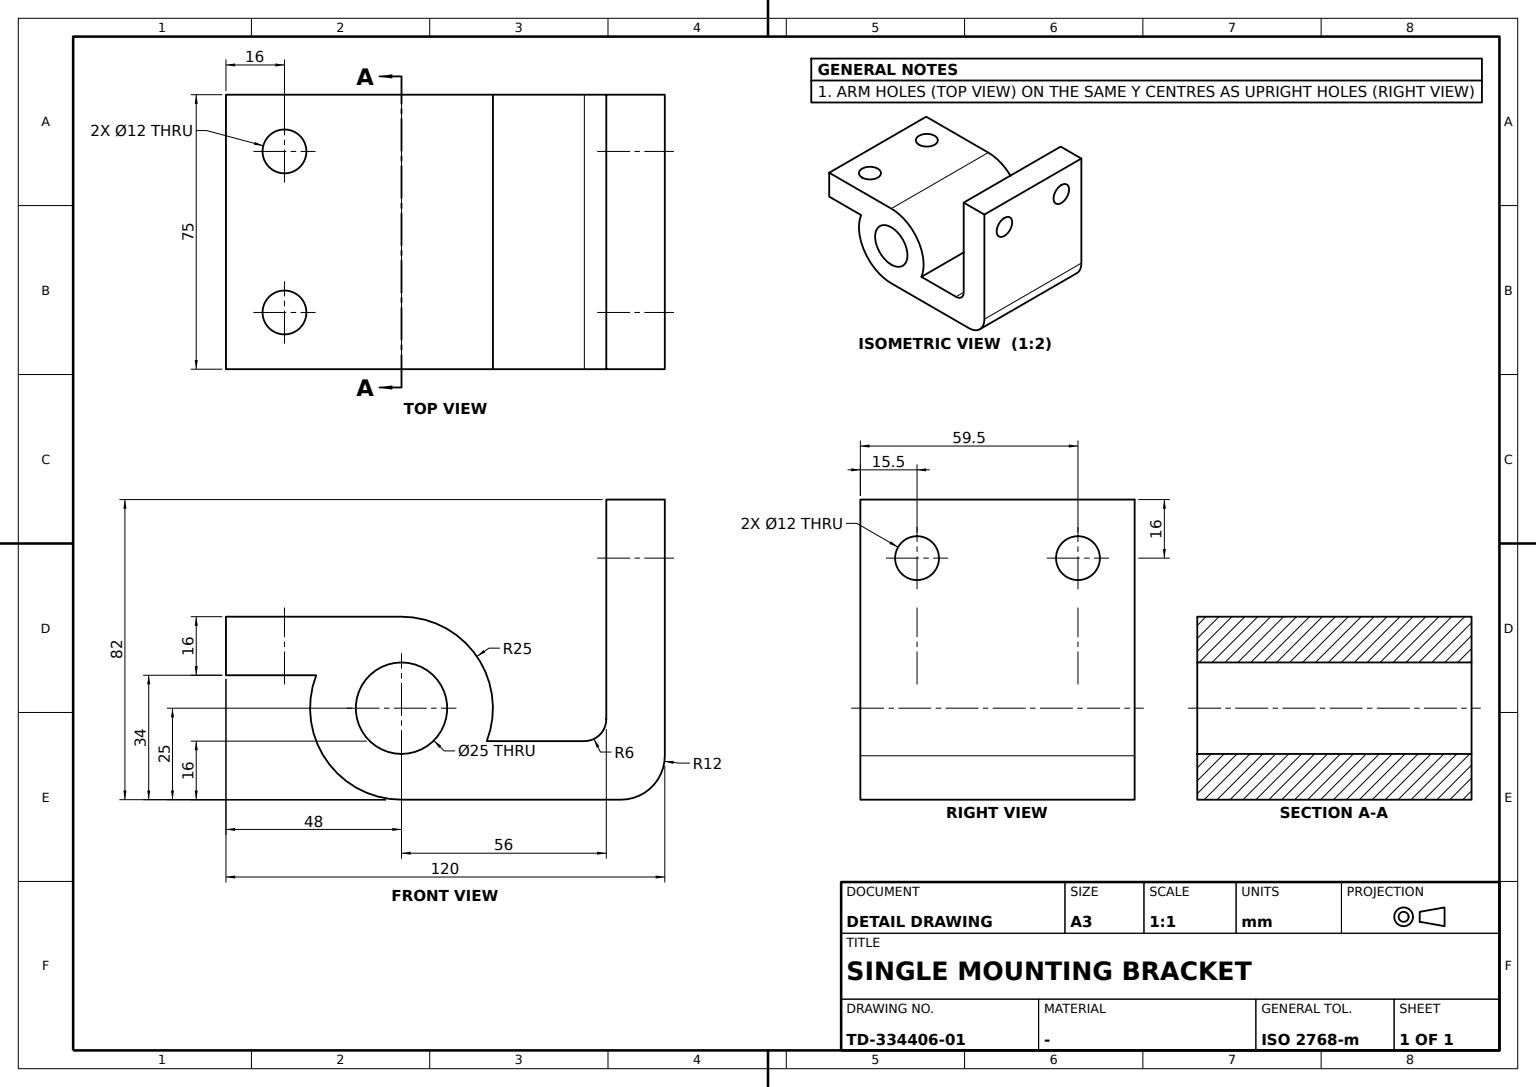
ISO-10303-21;
HEADER;
FILE_DESCRIPTION((''),'2;1');
FILE_NAME('','',(''),(''),'','','');
FILE_SCHEMA(('AUTOMOTIVE_DESIGN'));
ENDSEC;
DATA;
#1=APPLICATION_CONTEXT('');
#2=PRODUCT_CONTEXT('',#1,'mechanical');
#3=PRODUCT('','','',(#2));
#4=PRODUCT_DEFINITION_FORMATION('','',#3);
#5=PRODUCT_DEFINITION_CONTEXT('',#1,'design');
#6=PRODUCT_DEFINITION('','',#4,#5);
#7=PRODUCT_DEFINITION_SHAPE('','',#6);
#8=(LENGTH_UNIT()NAMED_UNIT(*)SI_UNIT(.MILLI.,.METRE.));
#9=(NAMED_UNIT(*)PLANE_ANGLE_UNIT()SI_UNIT($,.RADIAN.));
#10=(NAMED_UNIT(*)SI_UNIT($,.STERADIAN.)SOLID_ANGLE_UNIT());
#11=UNCERTAINTY_MEASURE_WITH_UNIT(LENGTH_MEASURE(0.005),#8,'distance_accuracy_value','');
#12=(GEOMETRIC_REPRESENTATION_CONTEXT(3)GLOBAL_UNCERTAINTY_ASSIGNED_CONTEXT((#11))GLOBAL_UNIT_ASSIGNED_CONTEXT((#8,#9,#10))REPRESENTATION_CONTEXT('',''));
#13=CARTESIAN_POINT('',(-37.5,-23.323808,9.));
#14=VERTEX_POINT('',#13);
#15=CARTESIAN_POINT('',(-37.5,0.,-25.));
#16=VERTEX_POINT('',#15);
#17=CARTESIAN_POINT('',(-37.5,0.,0.));
#18=DIRECTION('',(1.,0.,0.));
#19=DIRECTION('',(0.,0.,-1.));
#20=AXIS2_PLACEMENT_3D('',#17,#18,#19);
#21=CIRCLE('',#20,25.);
#22=EDGE_CURVE('',#14,#16,#21,.T.);
#23=ORIENTED_EDGE('',*,*,#22,.T.);
#24=CARTESIAN_POINT('',(37.5,0.,-25.));
#25=VERTEX_POINT('',#24);
#26=CARTESIAN_POINT('',(0.,0.,-25.));
#27=VECTOR('',#18,1000.);
#28=LINE('',#26,#27);
#29=EDGE_CURVE('',#16,#25,#28,.T.);
#30=ORIENTED_EDGE('',*,*,#29,.T.);
#31=CARTESIAN_POINT('',(37.5,-23.323808,9.));
#32=VERTEX_POINT('',#31);
#33=CARTESIAN_POINT('',(37.5,0.,0.));
#34=AXIS2_PLACEMENT_3D('',#33,#18,#19);
#35=CIRCLE('',#34,25.);
#36=EDGE_CURVE('',#32,#25,#35,.T.);
#37=ORIENTED_EDGE('',*,*,#36,.F.);
#38=LINE('',#13,#27);
#39=EDGE_CURVE('',#14,#32,#38,.T.);
#40=ORIENTED_EDGE('',*,*,#39,.F.);
#41=EDGE_LOOP('',(#23,#30,#37,#40));
#42=FACE_BOUND('',#41,.T.);
#43=CARTESIAN_POINT('',(0.,0.,0.));
#44=DIRECTION('',(0.,1.,0.));
#45=AXIS2_PLACEMENT_3D('',#43,#18,#44);
#46=CYLINDRICAL_SURFACE('',#45,25.);
#47=ADVANCED_FACE('',(#42),#46,.T.);
#48=CARTESIAN_POINT('',(22.,56.,47.));
#49=VERTEX_POINT('',#48);
#50=CARTESIAN_POINT('',(22.,56.,41.));
#51=DIRECTION('',(0.,0.,1.));
#52=AXIS2_PLACEMENT_3D('',#50,#44,#51);
#53=CIRCLE('',#52,6.);
#54=EDGE_CURVE('',#49,#49,#53,.T.);
#55=ORIENTED_EDGE('',*,*,#54,.F.);
#56=EDGE_LOOP('',(#55));
#57=FACE_BOUND('',#56,.T.);
#58=CARTESIAN_POINT('',(22.,72.,35.));
#59=VERTEX_POINT('',#58);
#60=CARTESIAN_POINT('',(22.,72.,41.));
#61=DIRECTION('',(0.,-1.,0.));
#62=AXIS2_PLACEMENT_3D('',#60,#61,#19);
#63=CIRCLE('',#62,6.);
#64=EDGE_CURVE('',#59,#59,#63,.F.);
#65=ORIENTED_EDGE('',*,*,#64,.T.);
#66=EDGE_LOOP('',(#65));
#67=FACE_BOUND('',#66,.T.);
#68=CARTESIAN_POINT('',(22.,53.25,41.));
#69=DIRECTION('',(-1.,0.,0.));
#70=AXIS2_PLACEMENT_3D('',#68,#44,#69);
#71=CYLINDRICAL_SURFACE('',#70,6.);
#72=ADVANCED_FACE('',(#57,#67),#71,.F.);
#73=CARTESIAN_POINT('',(-37.5,0.,25.));
#74=VERTEX_POINT('',#73);
#75=CARTESIAN_POINT('',(37.5,0.,25.));
#76=VERTEX_POINT('',#75);
#77=CARTESIAN_POINT('',(0.,0.,25.));
#78=LINE('',#77,#27);
#79=EDGE_CURVE('',#74,#76,#78,.T.);
#80=ORIENTED_EDGE('',*,*,#79,.T.);
#81=CARTESIAN_POINT('',(37.5,23.323808,-9.));
#82=VERTEX_POINT('',#81);
#83=EDGE_CURVE('',#82,#76,#35,.T.);
#84=ORIENTED_EDGE('',*,*,#83,.F.);
#85=CARTESIAN_POINT('',(-37.5,23.323808,-9.));
#86=VERTEX_POINT('',#85);
#87=LINE('',#85,#27);
#88=EDGE_CURVE('',#86,#82,#87,.T.);
#89=ORIENTED_EDGE('',*,*,#88,.F.);
#90=EDGE_CURVE('',#86,#74,#21,.T.);
#91=ORIENTED_EDGE('',*,*,#90,.T.);
#92=EDGE_LOOP('',(#80,#84,#89,#91));
#93=FACE_BOUND('',#92,.T.);
#94=ADVANCED_FACE('',(#93),#46,.T.);
#95=CARTESIAN_POINT('',(37.5,0.,-12.5));
#96=VERTEX_POINT('',#95);
#97=CIRCLE('',#34,12.5);
#98=EDGE_CURVE('',#96,#96,#97,.T.);
#99=ORIENTED_EDGE('',*,*,#98,.T.);
#100=EDGE_LOOP('',(#99));
#101=FACE_BOUND('',#100,.T.);
#102=CARTESIAN_POINT('',(-37.5,0.,-12.5));
#103=VERTEX_POINT('',#102);
#104=CIRCLE('',#20,12.5);
#105=EDGE_CURVE('',#103,#103,#104,.T.);
#106=ORIENTED_EDGE('',*,*,#105,.F.);
#107=EDGE_LOOP('',(#106));
#108=FACE_BOUND('',#107,.T.);
#109=CYLINDRICAL_SURFACE('',#45,12.5);
#110=ADVANCED_FACE('',(#101,#108),#109,.F.);
#111=CARTESIAN_POINT('',(16.,-32.,9.));
#112=VERTEX_POINT('',#111);
#113=CARTESIAN_POINT('',(22.,-32.,9.));
#114=AXIS2_PLACEMENT_3D('',#113,#19,#69);
#115=CIRCLE('',#114,6.);
#116=EDGE_CURVE('',#112,#112,#115,.T.);
#117=ORIENTED_EDGE('',*,*,#116,.F.);
#118=EDGE_LOOP('',(#117));
#119=FACE_BOUND('',#118,.T.);
#120=CARTESIAN_POINT('',(-28.,-32.,9.));
#121=VERTEX_POINT('',#120);
#122=CARTESIAN_POINT('',(-22.,-32.,9.));
#123=AXIS2_PLACEMENT_3D('',#122,#19,#69);
#124=CIRCLE('',#123,6.);
#125=EDGE_CURVE('',#121,#121,#124,.T.);
#126=ORIENTED_EDGE('',*,*,#125,.F.);
#127=EDGE_LOOP('',(#126));
#128=FACE_BOUND('',#127,.T.);
#129=CARTESIAN_POINT('',(37.5,-48.,9.));
#130=VERTEX_POINT('',#129);
#131=CARTESIAN_POINT('',(37.5,0.,9.));
#132=VECTOR('',#44,1000.);
#133=LINE('',#131,#132);
#134=EDGE_CURVE('',#130,#32,#133,.T.);
#135=ORIENTED_EDGE('',*,*,#134,.F.);
#136=CARTESIAN_POINT('',(-37.5,-48.,9.));
#137=VERTEX_POINT('',#136);
#138=CARTESIAN_POINT('',(0.,-48.,9.));
#139=LINE('',#138,#27);
#140=EDGE_CURVE('',#137,#130,#139,.T.);
#141=ORIENTED_EDGE('',*,*,#140,.F.);
#142=CARTESIAN_POINT('',(-37.5,0.,9.));
#143=LINE('',#142,#132);
#144=EDGE_CURVE('',#137,#14,#143,.T.);
#145=ORIENTED_EDGE('',*,*,#144,.T.);
#146=ORIENTED_EDGE('',*,*,#39,.T.);
#147=EDGE_LOOP('',(#135,#141,#145,#146));
#148=FACE_BOUND('',#147,.T.);
#149=AXIS2_PLACEMENT_3D('',#138,#19,#44);
#150=PLANE('',#149);
#151=ADVANCED_FACE('',(#119,#128,#148),#150,.T.);
#152=ORIENTED_EDGE('',*,*,#125,.T.);
#153=EDGE_LOOP('',(#152));
#154=FACE_BOUND('',#153,.T.);
#155=CARTESIAN_POINT('',(-16.,-32.,25.));
#156=VERTEX_POINT('',#155);
#157=CARTESIAN_POINT('',(-22.,-32.,25.));
#158=AXIS2_PLACEMENT_3D('',#157,#51,#18);
#159=CIRCLE('',#158,6.);
#160=EDGE_CURVE('',#156,#156,#159,.T.);
#161=ORIENTED_EDGE('',*,*,#160,.T.);
#162=EDGE_LOOP('',(#161));
#163=FACE_BOUND('',#162,.T.);
#164=CARTESIAN_POINT('',(-22.,-32.,6.25));
#165=AXIS2_PLACEMENT_3D('',#164,#51,#44);
#166=CYLINDRICAL_SURFACE('',#165,6.);
#167=ADVANCED_FACE('',(#154,#163),#166,.F.);
#168=CARTESIAN_POINT('',(-37.5,60.,-25.));
#169=VERTEX_POINT('',#168);
#170=CARTESIAN_POINT('',(37.5,60.,-25.));
#171=VERTEX_POINT('',#170);
#172=CARTESIAN_POINT('',(0.,60.,-25.));
#173=LINE('',#172,#27);
#174=EDGE_CURVE('',#169,#171,#173,.T.);
#175=ORIENTED_EDGE('',*,*,#174,.F.);
#176=CARTESIAN_POINT('',(-37.5,72.,-13.));
#177=VERTEX_POINT('',#176);
#178=CARTESIAN_POINT('',(-37.5,60.,-13.));
#179=AXIS2_PLACEMENT_3D('',#178,#18,#19);
#180=CIRCLE('',#179,12.);
#181=EDGE_CURVE('',#169,#177,#180,.T.);
#182=ORIENTED_EDGE('',*,*,#181,.T.);
#183=CARTESIAN_POINT('',(37.5,72.,-13.));
#184=VERTEX_POINT('',#183);
#185=CARTESIAN_POINT('',(0.,72.,-13.));
#186=LINE('',#185,#27);
#187=EDGE_CURVE('',#177,#184,#186,.T.);
#188=ORIENTED_EDGE('',*,*,#187,.T.);
#189=CARTESIAN_POINT('',(37.5,60.,-13.));
#190=AXIS2_PLACEMENT_3D('',#189,#18,#19);
#191=CIRCLE('',#190,12.);
#192=EDGE_CURVE('',#171,#184,#191,.T.);
#193=ORIENTED_EDGE('',*,*,#192,.F.);
#194=EDGE_LOOP('',(#175,#182,#188,#193));
#195=FACE_BOUND('',#194,.T.);
#196=CARTESIAN_POINT('',(0.,60.,-13.));
#197=AXIS2_PLACEMENT_3D('',#196,#18,#44);
#198=CYLINDRICAL_SURFACE('',#197,12.);
#199=ADVANCED_FACE('',(#195),#198,.T.);
#200=CARTESIAN_POINT('',(-22.,72.,35.));
#201=VERTEX_POINT('',#200);
#202=CARTESIAN_POINT('',(-22.,72.,41.));
#203=AXIS2_PLACEMENT_3D('',#202,#61,#19);
#204=CIRCLE('',#203,6.);
#205=EDGE_CURVE('',#201,#201,#204,.F.);
#206=ORIENTED_EDGE('',*,*,#205,.T.);
#207=EDGE_LOOP('',(#206));
#208=FACE_BOUND('',#207,.T.);
#209=CARTESIAN_POINT('',(-22.,56.,47.));
#210=VERTEX_POINT('',#209);
#211=CARTESIAN_POINT('',(-22.,56.,41.));
#212=AXIS2_PLACEMENT_3D('',#211,#44,#51);
#213=CIRCLE('',#212,6.);
#214=EDGE_CURVE('',#210,#210,#213,.T.);
#215=ORIENTED_EDGE('',*,*,#214,.F.);
#216=EDGE_LOOP('',(#215));
#217=FACE_BOUND('',#216,.T.);
#218=CARTESIAN_POINT('',(-22.,53.25,41.));
#219=AXIS2_PLACEMENT_3D('',#218,#44,#69);
#220=CYLINDRICAL_SURFACE('',#219,6.);
#221=ADVANCED_FACE('',(#208,#217),#220,.F.);
#222=ORIENTED_EDGE('',*,*,#144,.F.);
#223=CARTESIAN_POINT('',(-37.5,-48.,25.));
#224=VERTEX_POINT('',#223);
#225=CARTESIAN_POINT('',(-37.5,-48.,0.));
#226=VECTOR('',#19,1000.);
#227=LINE('',#225,#226);
#228=EDGE_CURVE('',#224,#137,#227,.T.);
#229=ORIENTED_EDGE('',*,*,#228,.F.);
#230=VECTOR('',#61,1000.);
#231=LINE('',#73,#230);
#232=EDGE_CURVE('',#74,#224,#231,.T.);
#233=ORIENTED_EDGE('',*,*,#232,.F.);
#234=ORIENTED_EDGE('',*,*,#90,.F.);
#235=CARTESIAN_POINT('',(-37.5,50.,-9.));
#236=VERTEX_POINT('',#235);
#237=CARTESIAN_POINT('',(-37.5,0.,-9.));
#238=LINE('',#237,#132);
#239=EDGE_CURVE('',#86,#236,#238,.T.);
#240=ORIENTED_EDGE('',*,*,#239,.T.);
#241=CARTESIAN_POINT('',(-37.5,56.,-3.));
#242=VERTEX_POINT('',#241);
#243=CARTESIAN_POINT('',(-37.5,50.,-3.));
#244=AXIS2_PLACEMENT_3D('',#243,#18,#19);
#245=CIRCLE('',#244,6.);
#246=EDGE_CURVE('',#236,#242,#245,.T.);
#247=ORIENTED_EDGE('',*,*,#246,.T.);
#248=CARTESIAN_POINT('',(-37.5,56.,57.));
#249=VERTEX_POINT('',#248);
#250=CARTESIAN_POINT('',(-37.5,56.,0.));
#251=VECTOR('',#51,1000.);
#252=LINE('',#250,#251);
#253=EDGE_CURVE('',#242,#249,#252,.T.);
#254=ORIENTED_EDGE('',*,*,#253,.T.);
#255=CARTESIAN_POINT('',(-37.5,72.,57.));
#256=VERTEX_POINT('',#255);
#257=CARTESIAN_POINT('',(-37.5,0.,57.));
#258=LINE('',#257,#132);
#259=EDGE_CURVE('',#249,#256,#258,.T.);
#260=ORIENTED_EDGE('',*,*,#259,.T.);
#261=CARTESIAN_POINT('',(-37.5,72.,0.));
#262=LINE('',#261,#226);
#263=EDGE_CURVE('',#256,#177,#262,.T.);
#264=ORIENTED_EDGE('',*,*,#263,.T.);
#265=ORIENTED_EDGE('',*,*,#181,.F.);
#266=LINE('',#15,#230);
#267=EDGE_CURVE('',#169,#16,#266,.T.);
#268=ORIENTED_EDGE('',*,*,#267,.T.);
#269=ORIENTED_EDGE('',*,*,#22,.F.);
#270=EDGE_LOOP('',(#222,#229,#233,#234,#240,#247,#254,#260,#264,#265,#268,#269));
#271=FACE_BOUND('',#270,.T.);
#272=ORIENTED_EDGE('',*,*,#105,.T.);
#273=EDGE_LOOP('',(#272));
#274=FACE_BOUND('',#273,.T.);
#275=AXIS2_PLACEMENT_3D('',#17,#18,#44);
#276=PLANE('',#275);
#277=ADVANCED_FACE('',(#271,#274),#276,.F.);
#278=CARTESIAN_POINT('',(28.,-32.,25.));
#279=VERTEX_POINT('',#278);
#280=CARTESIAN_POINT('',(22.,-32.,25.));
#281=AXIS2_PLACEMENT_3D('',#280,#51,#18);
#282=CIRCLE('',#281,6.);
#283=EDGE_CURVE('',#279,#279,#282,.T.);
#284=ORIENTED_EDGE('',*,*,#283,.T.);
#285=EDGE_LOOP('',(#284));
#286=FACE_BOUND('',#285,.T.);
#287=ORIENTED_EDGE('',*,*,#116,.T.);
#288=EDGE_LOOP('',(#287));
#289=FACE_BOUND('',#288,.T.);
#290=CARTESIAN_POINT('',(22.,-32.,6.25));
#291=AXIS2_PLACEMENT_3D('',#290,#51,#44);
#292=CYLINDRICAL_SURFACE('',#291,6.);
#293=ADVANCED_FACE('',(#286,#289),#292,.F.);
#294=CARTESIAN_POINT('',(37.5,56.,57.));
#295=VERTEX_POINT('',#294);
#296=CARTESIAN_POINT('',(37.5,72.,57.));
#297=VERTEX_POINT('',#296);
#298=CARTESIAN_POINT('',(37.5,0.,57.));
#299=LINE('',#298,#132);
#300=EDGE_CURVE('',#295,#297,#299,.T.);
#301=ORIENTED_EDGE('',*,*,#300,.T.);
#302=CARTESIAN_POINT('',(0.,72.,57.));
#303=LINE('',#302,#27);
#304=EDGE_CURVE('',#256,#297,#303,.T.);
#305=ORIENTED_EDGE('',*,*,#304,.F.);
#306=ORIENTED_EDGE('',*,*,#259,.F.);
#307=CARTESIAN_POINT('',(0.,56.,57.));
#308=LINE('',#307,#27);
#309=EDGE_CURVE('',#249,#295,#308,.T.);
#310=ORIENTED_EDGE('',*,*,#309,.T.);
#311=EDGE_LOOP('',(#301,#305,#306,#310));
#312=FACE_BOUND('',#311,.T.);
#313=AXIS2_PLACEMENT_3D('',#307,#19,#44);
#314=PLANE('',#313);
#315=ADVANCED_FACE('',(#312),#314,.F.);
#316=ORIENTED_EDGE('',*,*,#205,.F.);
#317=EDGE_LOOP('',(#316));
#318=FACE_BOUND('',#317,.T.);
#319=ORIENTED_EDGE('',*,*,#64,.F.);
#320=EDGE_LOOP('',(#319));
#321=FACE_BOUND('',#320,.T.);
#322=ORIENTED_EDGE('',*,*,#187,.F.);
#323=ORIENTED_EDGE('',*,*,#263,.F.);
#324=ORIENTED_EDGE('',*,*,#304,.T.);
#325=CARTESIAN_POINT('',(37.5,72.,0.));
#326=LINE('',#325,#226);
#327=EDGE_CURVE('',#297,#184,#326,.T.);
#328=ORIENTED_EDGE('',*,*,#327,.T.);
#329=EDGE_LOOP('',(#322,#323,#324,#328));
#330=FACE_BOUND('',#329,.T.);
#331=AXIS2_PLACEMENT_3D('',#302,#61,#19);
#332=PLANE('',#331);
#333=ADVANCED_FACE('',(#318,#321,#330),#332,.F.);
#334=ORIENTED_EDGE('',*,*,#98,.F.);
#335=EDGE_LOOP('',(#334));
#336=FACE_BOUND('',#335,.T.);
#337=LINE('',#24,#230);
#338=EDGE_CURVE('',#171,#25,#337,.T.);
#339=ORIENTED_EDGE('',*,*,#338,.F.);
#340=ORIENTED_EDGE('',*,*,#192,.T.);
#341=ORIENTED_EDGE('',*,*,#327,.F.);
#342=ORIENTED_EDGE('',*,*,#300,.F.);
#343=CARTESIAN_POINT('',(37.5,56.,-3.));
#344=VERTEX_POINT('',#343);
#345=CARTESIAN_POINT('',(37.5,56.,0.));
#346=LINE('',#345,#251);
#347=EDGE_CURVE('',#344,#295,#346,.T.);
#348=ORIENTED_EDGE('',*,*,#347,.F.);
#349=CARTESIAN_POINT('',(37.5,50.,-9.));
#350=VERTEX_POINT('',#349);
#351=CARTESIAN_POINT('',(37.5,50.,-3.));
#352=AXIS2_PLACEMENT_3D('',#351,#18,#19);
#353=CIRCLE('',#352,6.);
#354=EDGE_CURVE('',#350,#344,#353,.T.);
#355=ORIENTED_EDGE('',*,*,#354,.F.);
#356=CARTESIAN_POINT('',(37.5,0.,-9.));
#357=LINE('',#356,#132);
#358=EDGE_CURVE('',#82,#350,#357,.T.);
#359=ORIENTED_EDGE('',*,*,#358,.F.);
#360=ORIENTED_EDGE('',*,*,#83,.T.);
#361=CARTESIAN_POINT('',(37.5,-48.,25.));
#362=VERTEX_POINT('',#361);
#363=LINE('',#75,#230);
#364=EDGE_CURVE('',#76,#362,#363,.T.);
#365=ORIENTED_EDGE('',*,*,#364,.T.);
#366=CARTESIAN_POINT('',(37.5,-48.,0.));
#367=LINE('',#366,#226);
#368=EDGE_CURVE('',#362,#130,#367,.T.);
#369=ORIENTED_EDGE('',*,*,#368,.T.);
#370=ORIENTED_EDGE('',*,*,#134,.T.);
#371=ORIENTED_EDGE('',*,*,#36,.T.);
#372=EDGE_LOOP('',(#339,#340,#341,#342,#348,#355,#359,#360,#365,#369,#370,#371));
#373=FACE_BOUND('',#372,.T.);
#374=AXIS2_PLACEMENT_3D('',#33,#18,#44);
#375=PLANE('',#374);
#376=ADVANCED_FACE('',(#336,#373),#375,.T.);
#377=ORIENTED_EDGE('',*,*,#228,.T.);
#378=ORIENTED_EDGE('',*,*,#140,.T.);
#379=ORIENTED_EDGE('',*,*,#368,.F.);
#380=CARTESIAN_POINT('',(0.,-48.,25.));
#381=LINE('',#380,#27);
#382=EDGE_CURVE('',#224,#362,#381,.T.);
#383=ORIENTED_EDGE('',*,*,#382,.F.);
#384=EDGE_LOOP('',(#377,#378,#379,#383));
#385=FACE_BOUND('',#384,.T.);
#386=AXIS2_PLACEMENT_3D('',#380,#61,#19);
#387=PLANE('',#386);
#388=ADVANCED_FACE('',(#385),#387,.T.);
#389=ORIENTED_EDGE('',*,*,#29,.F.);
#390=ORIENTED_EDGE('',*,*,#267,.F.);
#391=ORIENTED_EDGE('',*,*,#174,.T.);
#392=ORIENTED_EDGE('',*,*,#338,.T.);
#393=EDGE_LOOP('',(#389,#390,#391,#392));
#394=FACE_BOUND('',#393,.T.);
#395=CARTESIAN_POINT('',(0.,72.,-25.));
#396=AXIS2_PLACEMENT_3D('',#395,#51,#61);
#397=PLANE('',#396);
#398=ADVANCED_FACE('',(#394),#397,.F.);
#399=ORIENTED_EDGE('',*,*,#214,.T.);
#400=EDGE_LOOP('',(#399));
#401=FACE_BOUND('',#400,.T.);
#402=ORIENTED_EDGE('',*,*,#253,.F.);
#403=CARTESIAN_POINT('',(0.,56.,-3.));
#404=LINE('',#403,#27);
#405=EDGE_CURVE('',#242,#344,#404,.T.);
#406=ORIENTED_EDGE('',*,*,#405,.T.);
#407=ORIENTED_EDGE('',*,*,#347,.T.);
#408=ORIENTED_EDGE('',*,*,#309,.F.);
#409=EDGE_LOOP('',(#402,#406,#407,#408));
#410=FACE_BOUND('',#409,.T.);
#411=ORIENTED_EDGE('',*,*,#54,.T.);
#412=EDGE_LOOP('',(#411));
#413=FACE_BOUND('',#412,.T.);
#414=CARTESIAN_POINT('',(0.,56.,-9.));
#415=AXIS2_PLACEMENT_3D('',#414,#44,#51);
#416=PLANE('',#415);
#417=ADVANCED_FACE('',(#401,#410,#413),#416,.F.);
#418=ORIENTED_EDGE('',*,*,#354,.T.);
#419=ORIENTED_EDGE('',*,*,#405,.F.);
#420=ORIENTED_EDGE('',*,*,#246,.F.);
#421=CARTESIAN_POINT('',(0.,50.,-9.));
#422=LINE('',#421,#27);
#423=EDGE_CURVE('',#236,#350,#422,.T.);
#424=ORIENTED_EDGE('',*,*,#423,.T.);
#425=EDGE_LOOP('',(#418,#419,#420,#424));
#426=FACE_BOUND('',#425,.T.);
#427=CARTESIAN_POINT('',(0.,50.,-3.));
#428=AXIS2_PLACEMENT_3D('',#427,#18,#19);
#429=CYLINDRICAL_SURFACE('',#428,6.);
#430=ADVANCED_FACE('',(#426),#429,.F.);
#431=ORIENTED_EDGE('',*,*,#283,.F.);
#432=EDGE_LOOP('',(#431));
#433=FACE_BOUND('',#432,.T.);
#434=ORIENTED_EDGE('',*,*,#160,.F.);
#435=EDGE_LOOP('',(#434));
#436=FACE_BOUND('',#435,.T.);
#437=ORIENTED_EDGE('',*,*,#382,.T.);
#438=ORIENTED_EDGE('',*,*,#364,.F.);
#439=ORIENTED_EDGE('',*,*,#79,.F.);
#440=ORIENTED_EDGE('',*,*,#232,.T.);
#441=EDGE_LOOP('',(#437,#438,#439,#440));
#442=FACE_BOUND('',#441,.T.);
#443=AXIS2_PLACEMENT_3D('',#77,#51,#61);
#444=PLANE('',#443);
#445=ADVANCED_FACE('',(#433,#436,#442),#444,.T.);
#446=ORIENTED_EDGE('',*,*,#239,.F.);
#447=ORIENTED_EDGE('',*,*,#88,.T.);
#448=ORIENTED_EDGE('',*,*,#358,.T.);
#449=ORIENTED_EDGE('',*,*,#423,.F.);
#450=EDGE_LOOP('',(#446,#447,#448,#449));
#451=FACE_BOUND('',#450,.T.);
#452=CARTESIAN_POINT('',(0.,23.323808,-9.));
#453=AXIS2_PLACEMENT_3D('',#452,#19,#44);
#454=PLANE('',#453);
#455=ADVANCED_FACE('',(#451),#454,.F.);
#456=CLOSED_SHELL('',(#47,#72,#94,#110,#151,#167,#199,#221,#277,#293,#315,#333,#376,#388,#398,#417,#430,#445,#455));
#457=MANIFOLD_SOLID_BREP('',#456);
#458=ADVANCED_BREP_SHAPE_REPRESENTATION('',(#457),#12);
#459=SHAPE_DEFINITION_REPRESENTATION(#7,#458);
ENDSEC;
END-ISO-10303-21;
